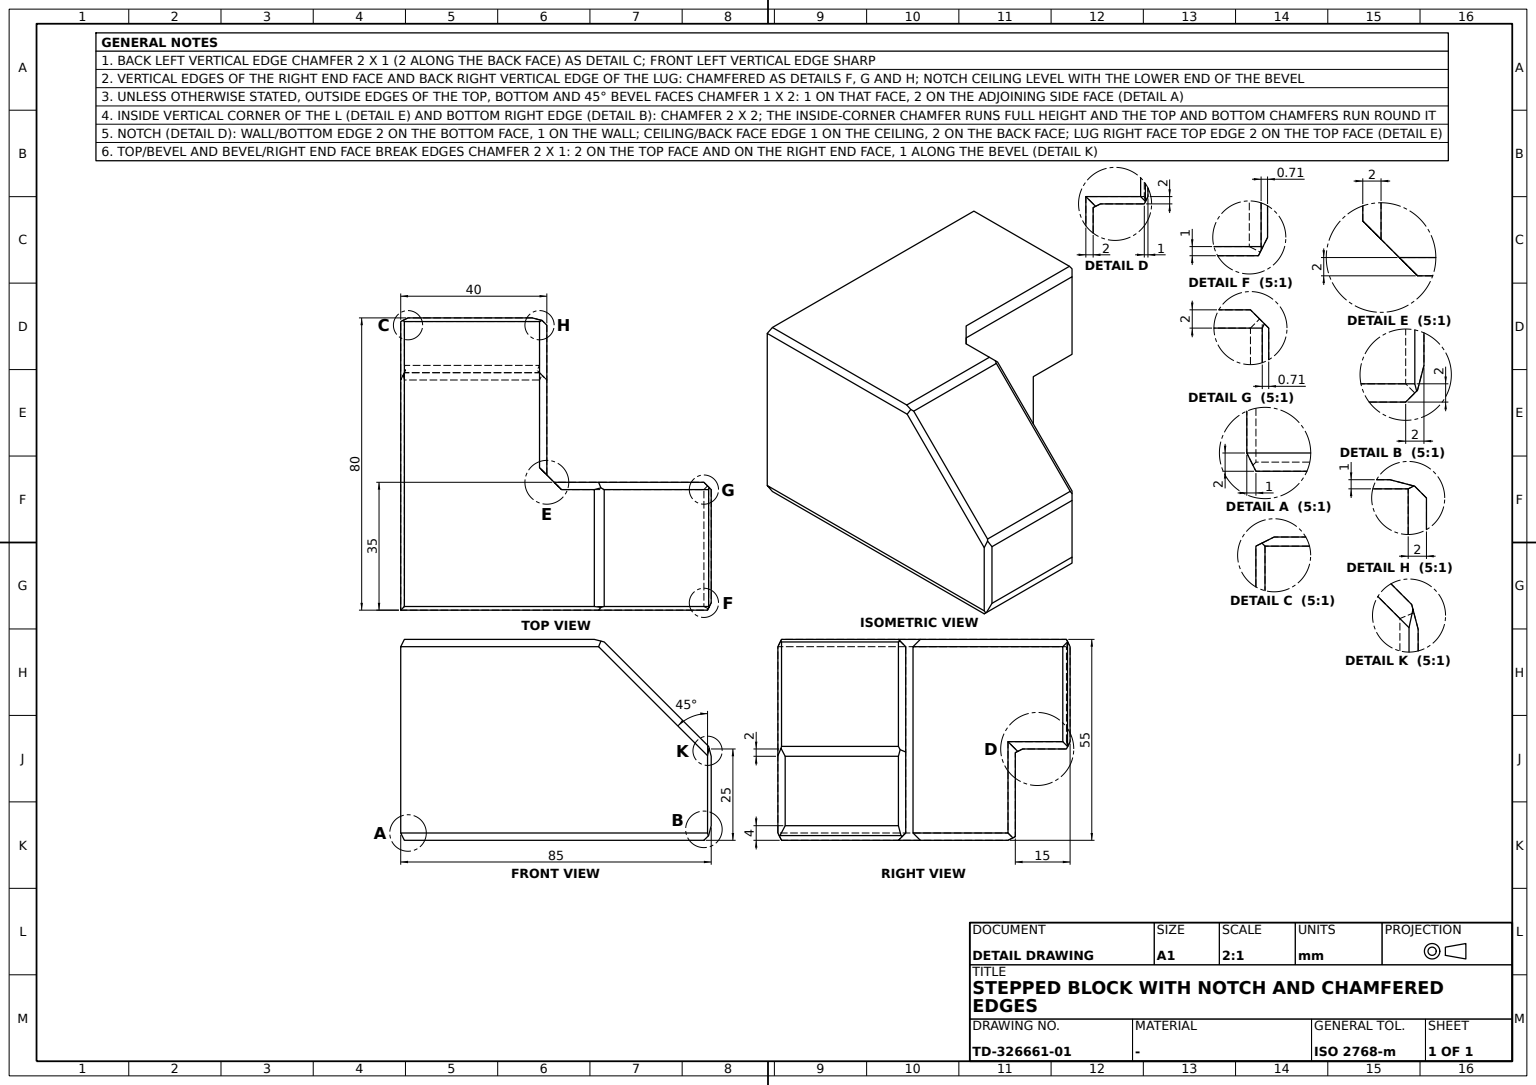
ISO-10303-21;
HEADER;
FILE_DESCRIPTION((''),'2;1');
FILE_NAME('','',(''),(''),'','','');
FILE_SCHEMA(('AUTOMOTIVE_DESIGN'));
ENDSEC;
DATA;
#1=APPLICATION_CONTEXT('');
#2=PRODUCT_CONTEXT('',#1,'mechanical');
#3=PRODUCT('','','',(#2));
#4=PRODUCT_DEFINITION_FORMATION('','',#3);
#5=PRODUCT_DEFINITION_CONTEXT('',#1,'design');
#6=PRODUCT_DEFINITION('','',#4,#5);
#7=PRODUCT_DEFINITION_SHAPE('','',#6);
#8=(LENGTH_UNIT()NAMED_UNIT(*)SI_UNIT(.MILLI.,.METRE.));
#9=(NAMED_UNIT(*)PLANE_ANGLE_UNIT()SI_UNIT($,.RADIAN.));
#10=(NAMED_UNIT(*)SI_UNIT($,.STERADIAN.)SOLID_ANGLE_UNIT());
#11=UNCERTAINTY_MEASURE_WITH_UNIT(LENGTH_MEASURE(0.005),#8,'distance_accuracy_value','');
#12=(GEOMETRIC_REPRESENTATION_CONTEXT(3)GLOBAL_UNCERTAINTY_ASSIGNED_CONTEXT((#11))GLOBAL_UNIT_ASSIGNED_CONTEXT((#8,#9,#10))REPRESENTATION_CONTEXT('',''));
#13=CARTESIAN_POINT('',(-42.5,-80.,53.));
#14=VERTEX_POINT('',#13);
#15=CARTESIAN_POINT('',(-41.5,-79.,55.));
#16=VERTEX_POINT('',#15);
#17=CARTESIAN_POINT('',(-45.166667,-82.666667,47.666667));
#18=DIRECTION('',(0.40824829,0.40824829,0.816496581));
#19=VECTOR('',#18,1000.);
#20=LINE('',#17,#19);
#21=EDGE_CURVE('',#14,#16,#20,.T.);
#22=ORIENTED_EDGE('',*,*,#21,.T.);
#23=CARTESIAN_POINT('',(-41.5,-1.,55.));
#24=VERTEX_POINT('',#23);
#25=CARTESIAN_POINT('',(-41.5,0.,55.));
#26=DIRECTION('',(0.,1.,0.));
#27=VECTOR('',#26,1000.);
#28=LINE('',#25,#27);
#29=EDGE_CURVE('',#16,#24,#28,.T.);
#30=ORIENTED_EDGE('',*,*,#29,.T.);
#31=CARTESIAN_POINT('',(-41.833333,-0.666667,54.333333));
#32=VERTEX_POINT('',#31);
#33=CARTESIAN_POINT('',(-44.066667,1.566667,49.866667));
#34=DIRECTION('',(0.40824829,-0.40824829,0.816496581));
#35=VECTOR('',#34,1000.);
#36=LINE('',#33,#35);
#37=EDGE_CURVE('',#32,#24,#36,.T.);
#38=ORIENTED_EDGE('',*,*,#37,.F.);
#39=CARTESIAN_POINT('',(-42.5,-1.,53.));
#40=VERTEX_POINT('',#39);
#41=CARTESIAN_POINT('',(-66.252381,-12.87619,5.495238));
#42=DIRECTION('',(0.43643578,0.21821789,0.872871561));
#43=VECTOR('',#42,1000.);
#44=LINE('',#41,#43);
#45=EDGE_CURVE('',#40,#32,#44,.T.);
#46=ORIENTED_EDGE('',*,*,#45,.F.);
#47=CARTESIAN_POINT('',(-42.5,-96.,53.));
#48=LINE('',#47,#27);
#49=EDGE_CURVE('',#14,#40,#48,.T.);
#50=ORIENTED_EDGE('',*,*,#49,.F.);
#51=EDGE_LOOP('',(#22,#30,#38,#46,#50));
#52=FACE_BOUND('',#51,.T.);
#53=DIRECTION('',(0.894427191,0.,-0.447213595));
#54=AXIS2_PLACEMENT_3D('',#47,#53,#26);
#55=PLANE('',#54);
#56=ADVANCED_FACE('',(#52),#55,.F.);
#57=CARTESIAN_POINT('',(13.207107,-47.,54.292893));
#58=VERTEX_POINT('',#57);
#59=CARTESIAN_POINT('',(13.207107,-79.,54.292893));
#60=VERTEX_POINT('',#59);
#61=CARTESIAN_POINT('',(13.207107,16.,54.292893));
#62=DIRECTION('',(0.,-1.,0.));
#63=VECTOR('',#62,1000.);
#64=LINE('',#61,#63);
#65=EDGE_CURVE('',#58,#60,#64,.T.);
#66=ORIENTED_EDGE('',*,*,#65,.F.);
#67=CARTESIAN_POINT('',(12.304738,-46.528595,54.528595));
#68=VERTEX_POINT('',#67);
#69=CARTESIAN_POINT('',(-13.48926,-33.053611,61.266088));
#70=DIRECTION('',(-0.863502056,0.451100166,0.225550083));
#71=VECTOR('',#70,1000.);
#72=LINE('',#69,#71);
#73=EDGE_CURVE('',#58,#68,#72,.T.);
#74=ORIENTED_EDGE('',*,*,#73,.T.);
#75=CARTESIAN_POINT('',(10.5,-47.,55.));
#76=VERTEX_POINT('',#75);
#77=CARTESIAN_POINT('',(24.97998,-43.217773,51.217773));
#78=DIRECTION('',(0.938045473,0.245021112,-0.245021112));
#79=VECTOR('',#78,1000.);
#80=LINE('',#77,#79);
#81=EDGE_CURVE('',#76,#68,#80,.T.);
#82=ORIENTED_EDGE('',*,*,#81,.F.);
#83=CARTESIAN_POINT('',(10.5,-79.,55.));
#84=VERTEX_POINT('',#83);
#85=CARTESIAN_POINT('',(10.5,16.,55.));
#86=LINE('',#85,#63);
#87=EDGE_CURVE('',#76,#84,#86,.T.);
#88=ORIENTED_EDGE('',*,*,#87,.T.);
#89=CARTESIAN_POINT('',(12.304738,-79.235702,54.528595));
#90=VERTEX_POINT('',#89);
#91=CARTESIAN_POINT('',(55.145452,-84.830783,43.338435));
#92=DIRECTION('',(0.959904955,-0.125365447,-0.250730894));
#93=VECTOR('',#92,1000.);
#94=LINE('',#91,#93);
#95=EDGE_CURVE('',#84,#90,#94,.T.);
#96=ORIENTED_EDGE('',*,*,#95,.T.);
#97=CARTESIAN_POINT('',(-2.503749,-83.103736,58.39663));
#98=DIRECTION('',(-0.938045473,-0.245021112,0.245021112));
#99=VECTOR('',#98,1000.);
#100=LINE('',#97,#99);
#101=EDGE_CURVE('',#60,#90,#100,.T.);
#102=ORIENTED_EDGE('',*,*,#101,.F.);
#103=EDGE_LOOP('',(#66,#74,#82,#88,#96,#102));
#104=FACE_BOUND('',#103,.T.);
#105=DIRECTION('',(0.252724733,0.,0.967538221));
#106=AXIS2_PLACEMENT_3D('',#85,#105,#62);
#107=PLANE('',#106);
#108=ADVANCED_FACE('',(#104),#107,.T.);
#109=CARTESIAN_POINT('',(-41.5,-17.,0.));
#110=VERTEX_POINT('',#109);
#111=CARTESIAN_POINT('',(-41.833333,-15.666667,0.666667));
#112=VERTEX_POINT('',#111);
#113=CARTESIAN_POINT('',(-36.804762,-35.780952,-9.390476));
#114=DIRECTION('',(-0.21821789,0.872871561,0.43643578));
#115=VECTOR('',#114,1000.);
#116=LINE('',#113,#115);
#117=EDGE_CURVE('',#110,#112,#116,.T.);
#118=ORIENTED_EDGE('',*,*,#117,.F.);
#119=CARTESIAN_POINT('',(-41.5,-79.,0.));
#120=VERTEX_POINT('',#119);
#121=CARTESIAN_POINT('',(-41.5,-95.8,0.));
#122=LINE('',#121,#27);
#123=EDGE_CURVE('',#120,#110,#122,.T.);
#124=ORIENTED_EDGE('',*,*,#123,.F.);
#125=CARTESIAN_POINT('',(-42.5,-80.,2.));
#126=VERTEX_POINT('',#125);
#127=CARTESIAN_POINT('',(-45.133333,-82.633333,7.266667));
#128=DIRECTION('',(-0.40824829,-0.40824829,0.816496581));
#129=VECTOR('',#128,1000.);
#130=LINE('',#127,#129);
#131=EDGE_CURVE('',#120,#126,#130,.T.);
#132=ORIENTED_EDGE('',*,*,#131,.T.);
#133=CARTESIAN_POINT('',(-42.5,-17.,2.));
#134=VERTEX_POINT('',#133);
#135=CARTESIAN_POINT('',(-42.5,-95.8,2.));
#136=LINE('',#135,#27);
#137=EDGE_CURVE('',#126,#134,#136,.T.);
#138=ORIENTED_EDGE('',*,*,#137,.T.);
#139=CARTESIAN_POINT('',(-60.011111,-52.022222,37.022222));
#140=DIRECTION('',(-0.333333333,-0.666666667,0.666666667));
#141=VECTOR('',#140,1000.);
#142=LINE('',#139,#141);
#143=EDGE_CURVE('',#112,#134,#142,.T.);
#144=ORIENTED_EDGE('',*,*,#143,.F.);
#145=EDGE_LOOP('',(#118,#124,#132,#138,#144));
#146=FACE_BOUND('',#145,.T.);
#147=DIRECTION('',(-0.894427191,0.,-0.447213595));
#148=AXIS2_PLACEMENT_3D('',#135,#147,#26);
#149=PLANE('',#148);
#150=ADVANCED_FACE('',(#146),#149,.T.);
#151=CARTESIAN_POINT('',(-41.833333,-0.666667,25.666667));
#152=VERTEX_POINT('',#151);
#153=CARTESIAN_POINT('',(-41.5,-1.,25.));
#154=VERTEX_POINT('',#153);
#155=CARTESIAN_POINT('',(-26.533333,-15.966667,-4.933333));
#156=DIRECTION('',(0.40824829,-0.40824829,-0.816496581));
#157=VECTOR('',#156,1000.);
#158=LINE('',#155,#157);
#159=EDGE_CURVE('',#152,#154,#158,.T.);
#160=ORIENTED_EDGE('',*,*,#159,.T.);
#161=CARTESIAN_POINT('',(-41.5,-13.,25.));
#162=VERTEX_POINT('',#161);
#163=CARTESIAN_POINT('',(-41.5,-95.8,25.));
#164=LINE('',#163,#27);
#165=EDGE_CURVE('',#162,#154,#164,.T.);
#166=ORIENTED_EDGE('',*,*,#165,.F.);
#167=CARTESIAN_POINT('',(-41.166667,-14.333333,24.333333));
#168=VERTEX_POINT('',#167);
#169=CARTESIAN_POINT('',(-25.966667,-75.133333,-6.066667));
#170=LINE('',#169,#115);
#171=EDGE_CURVE('',#168,#162,#170,.T.);
#172=ORIENTED_EDGE('',*,*,#171,.F.);
#173=CARTESIAN_POINT('',(-42.5,-17.,27.));
#174=VERTEX_POINT('',#173);
#175=CARTESIAN_POINT('',(-60.011111,-52.022222,62.022222));
#176=LINE('',#175,#141);
#177=EDGE_CURVE('',#168,#174,#176,.T.);
#178=ORIENTED_EDGE('',*,*,#177,.T.);
#179=CARTESIAN_POINT('',(-42.5,-1.,27.));
#180=VERTEX_POINT('',#179);
#181=CARTESIAN_POINT('',(-42.5,-95.8,27.));
#182=LINE('',#181,#27);
#183=EDGE_CURVE('',#174,#180,#182,.T.);
#184=ORIENTED_EDGE('',*,*,#183,.T.);
#185=CARTESIAN_POINT('',(-51.528571,-5.514286,45.057143));
#186=DIRECTION('',(-0.43643578,-0.21821789,0.872871561));
#187=VECTOR('',#186,1000.);
#188=LINE('',#185,#187);
#189=EDGE_CURVE('',#152,#180,#188,.T.);
#190=ORIENTED_EDGE('',*,*,#189,.F.);
#191=EDGE_LOOP('',(#160,#166,#172,#178,#184,#190));
#192=FACE_BOUND('',#191,.T.);
#193=AXIS2_PLACEMENT_3D('',#181,#147,#26);
#194=PLANE('',#193);
#195=ADVANCED_FACE('',(#192),#194,.T.);
#196=CARTESIAN_POINT('',(-40.5,0.,53.));
#197=VERTEX_POINT('',#196);
#198=CARTESIAN_POINT('',(-6.5,0.,53.));
#199=VERTEX_POINT('',#198);
#200=CARTESIAN_POINT('',(-51.9,0.,53.));
#201=DIRECTION('',(1.,0.,0.));
#202=VECTOR('',#201,1000.);
#203=LINE('',#200,#202);
#204=EDGE_CURVE('',#197,#199,#203,.T.);
#205=ORIENTED_EDGE('',*,*,#204,.T.);
#206=CARTESIAN_POINT('',(-6.5,0.,27.));
#207=VERTEX_POINT('',#206);
#208=CARTESIAN_POINT('',(-6.5,0.,19.933333));
#209=DIRECTION('',(0.,0.,1.));
#210=VECTOR('',#209,1000.);
#211=LINE('',#208,#210);
#212=EDGE_CURVE('',#207,#199,#211,.T.);
#213=ORIENTED_EDGE('',*,*,#212,.F.);
#214=CARTESIAN_POINT('',(-40.5,0.,27.));
#215=VERTEX_POINT('',#214);
#216=CARTESIAN_POINT('',(-50.1,0.,27.));
#217=LINE('',#216,#202);
#218=EDGE_CURVE('',#215,#207,#217,.T.);
#219=ORIENTED_EDGE('',*,*,#218,.F.);
#220=CARTESIAN_POINT('',(-40.5,0.,-10.6));
#221=LINE('',#220,#210);
#222=EDGE_CURVE('',#215,#197,#221,.T.);
#223=ORIENTED_EDGE('',*,*,#222,.T.);
#224=EDGE_LOOP('',(#205,#213,#219,#223));
#225=FACE_BOUND('',#224,.T.);
#226=CARTESIAN_POINT('',(-2.5,0.,0.));
#227=DIRECTION('',(-1.,0.,0.));
#228=AXIS2_PLACEMENT_3D('',#226,#26,#227);
#229=PLANE('',#228);
#230=ADVANCED_FACE('',(#225),#229,.T.);
#231=CARTESIAN_POINT('',(-41.5,-15.,24.));
#232=VERTEX_POINT('',#231);
#233=CARTESIAN_POINT('',(-33.266667,1.466667,32.233333));
#234=DIRECTION('',(0.40824829,0.816496581,0.40824829));
#235=VECTOR('',#234,1000.);
#236=LINE('',#233,#235);
#237=EDGE_CURVE('',#232,#168,#236,.T.);
#238=ORIENTED_EDGE('',*,*,#237,.T.);
#239=ORIENTED_EDGE('',*,*,#171,.T.);
#240=CARTESIAN_POINT('',(-4.5,-13.,25.));
#241=VERTEX_POINT('',#240);
#242=CARTESIAN_POINT('',(2.9,-13.,25.));
#243=VECTOR('',#227,1000.);
#244=LINE('',#242,#243);
#245=EDGE_CURVE('',#241,#162,#244,.T.);
#246=ORIENTED_EDGE('',*,*,#245,.F.);
#247=CARTESIAN_POINT('',(-5.166667,-14.333333,24.333333));
#248=VERTEX_POINT('',#247);
#249=CARTESIAN_POINT('',(-3.266667,-10.533333,26.233333));
#250=LINE('',#249,#235);
#251=EDGE_CURVE('',#248,#241,#250,.T.);
#252=ORIENTED_EDGE('',*,*,#251,.F.);
#253=CARTESIAN_POINT('',(-4.5,-15.,24.));
#254=VERTEX_POINT('',#253);
#255=CARTESIAN_POINT('',(-13.3,-6.2,28.4));
#256=DIRECTION('',(-0.666666667,0.666666667,0.333333333));
#257=VECTOR('',#256,1000.);
#258=LINE('',#255,#257);
#259=EDGE_CURVE('',#254,#248,#258,.T.);
#260=ORIENTED_EDGE('',*,*,#259,.F.);
#261=CARTESIAN_POINT('',(2.9,-15.,24.));
#262=LINE('',#261,#243);
#263=EDGE_CURVE('',#254,#232,#262,.T.);
#264=ORIENTED_EDGE('',*,*,#263,.T.);
#265=EDGE_LOOP('',(#238,#239,#246,#252,#260,#264));
#266=FACE_BOUND('',#265,.T.);
#267=DIRECTION('',(0.,-0.447213595,0.894427191));
#268=AXIS2_PLACEMENT_3D('',#242,#267,#227);
#269=PLANE('',#268);
#270=ADVANCED_FACE('',(#266),#269,.F.);
#271=CARTESIAN_POINT('',(-2.5,-2.,53.));
#272=VERTEX_POINT('',#271);
#273=CARTESIAN_POINT('',(-2.5,-43.,53.));
#274=VERTEX_POINT('',#273);
#275=CARTESIAN_POINT('',(-2.5,16.,53.));
#276=LINE('',#275,#63);
#277=EDGE_CURVE('',#272,#274,#276,.T.);
#278=ORIENTED_EDGE('',*,*,#277,.T.);
#279=CARTESIAN_POINT('',(-2.5,-43.,2.));
#280=VERTEX_POINT('',#279);
#281=CARTESIAN_POINT('',(-2.5,-43.,0.));
#282=LINE('',#281,#210);
#283=EDGE_CURVE('',#280,#274,#282,.T.);
#284=ORIENTED_EDGE('',*,*,#283,.F.);
#285=CARTESIAN_POINT('',(-2.5,-17.,2.));
#286=VERTEX_POINT('',#285);
#287=CARTESIAN_POINT('',(-2.5,-45.,2.));
#288=LINE('',#287,#27);
#289=EDGE_CURVE('',#280,#286,#288,.T.);
#290=ORIENTED_EDGE('',*,*,#289,.T.);
#291=CARTESIAN_POINT('',(-2.5,-17.,27.));
#292=VERTEX_POINT('',#291);
#293=CARTESIAN_POINT('',(-2.5,-17.,0.));
#294=DIRECTION('',(0.,0.,-1.));
#295=VECTOR('',#294,1000.);
#296=LINE('',#293,#295);
#297=EDGE_CURVE('',#292,#286,#296,.T.);
#298=ORIENTED_EDGE('',*,*,#297,.F.);
#299=CARTESIAN_POINT('',(-2.5,-2.,27.));
#300=VERTEX_POINT('',#299);
#301=CARTESIAN_POINT('',(-2.5,-45.,27.));
#302=LINE('',#301,#27);
#303=EDGE_CURVE('',#292,#300,#302,.T.);
#304=ORIENTED_EDGE('',*,*,#303,.T.);
#305=CARTESIAN_POINT('',(-2.5,-2.,0.));
#306=LINE('',#305,#295);
#307=EDGE_CURVE('',#272,#300,#306,.T.);
#308=ORIENTED_EDGE('',*,*,#307,.F.);
#309=EDGE_LOOP('',(#278,#284,#290,#298,#304,#308));
#310=FACE_BOUND('',#309,.T.);
#311=CARTESIAN_POINT('',(-2.5,-45.,0.));
#312=AXIS2_PLACEMENT_3D('',#311,#201,#26);
#313=PLANE('',#312);
#314=ADVANCED_FACE('',(#310),#313,.T.);
#315=CARTESIAN_POINT('',(-4.5,-41.,55.));
#316=VERTEX_POINT('',#315);
#317=CARTESIAN_POINT('',(1.5,-47.,55.));
#318=VERTEX_POINT('',#317);
#319=CARTESIAN_POINT('',(-2.5,-43.,55.));
#320=DIRECTION('',(0.707106781,-0.707106781,0.));
#321=VECTOR('',#320,1000.);
#322=LINE('',#319,#321);
#323=EDGE_CURVE('',#316,#318,#322,.T.);
#324=ORIENTED_EDGE('',*,*,#323,.F.);
#325=CARTESIAN_POINT('',(-4.5,-1.,55.));
#326=VERTEX_POINT('',#325);
#327=CARTESIAN_POINT('',(-4.5,0.,55.));
#328=LINE('',#327,#63);
#329=EDGE_CURVE('',#326,#316,#328,.T.);
#330=ORIENTED_EDGE('',*,*,#329,.F.);
#331=CARTESIAN_POINT('',(0.,-1.,55.));
#332=LINE('',#331,#202);
#333=EDGE_CURVE('',#24,#326,#332,.T.);
#334=ORIENTED_EDGE('',*,*,#333,.F.);
#335=ORIENTED_EDGE('',*,*,#29,.F.);
#336=CARTESIAN_POINT('',(0.,-79.,55.));
#337=LINE('',#336,#243);
#338=EDGE_CURVE('',#84,#16,#337,.T.);
#339=ORIENTED_EDGE('',*,*,#338,.F.);
#340=ORIENTED_EDGE('',*,*,#87,.F.);
#341=CARTESIAN_POINT('',(0.,-47.,55.));
#342=LINE('',#341,#202);
#343=EDGE_CURVE('',#318,#76,#342,.T.);
#344=ORIENTED_EDGE('',*,*,#343,.F.);
#345=EDGE_LOOP('',(#324,#330,#334,#335,#339,#340,#344));
#346=FACE_BOUND('',#345,.T.);
#347=CARTESIAN_POINT('',(0.,0.,55.));
#348=AXIS2_PLACEMENT_3D('',#347,#209,#201);
#349=PLANE('',#348);
#350=ADVANCED_FACE('',(#346),#349,.T.);
#351=CARTESIAN_POINT('',(40.5,-79.,0.));
#352=VERTEX_POINT('',#351);
#353=CARTESIAN_POINT('',(40.5,-47.,0.));
#354=VERTEX_POINT('',#353);
#355=CARTESIAN_POINT('',(40.5,0.,0.));
#356=LINE('',#355,#27);
#357=EDGE_CURVE('',#352,#354,#356,.T.);
#358=ORIENTED_EDGE('',*,*,#357,.T.);
#359=CARTESIAN_POINT('',(41.5,-46.,1.));
#360=VERTEX_POINT('',#359);
#361=CARTESIAN_POINT('',(46.833333,-40.666667,6.333333));
#362=DIRECTION('',(-0.577350269,-0.577350269,-0.577350269));
#363=VECTOR('',#362,1000.);
#364=LINE('',#361,#363);
#365=EDGE_CURVE('',#360,#354,#364,.T.);
#366=ORIENTED_EDGE('',*,*,#365,.F.);
#367=CARTESIAN_POINT('',(41.792893,-46.292893,1.292893));
#368=VERTEX_POINT('',#367);
#369=CARTESIAN_POINT('',(62.366667,-66.866667,21.866667));
#370=DIRECTION('',(0.577350269,-0.577350269,0.577350269));
#371=VECTOR('',#370,1000.);
#372=LINE('',#369,#371);
#373=EDGE_CURVE('',#360,#368,#372,.T.);
#374=ORIENTED_EDGE('',*,*,#373,.T.);
#375=CARTESIAN_POINT('',(41.792893,-79.414214,1.292893));
#376=VERTEX_POINT('',#375);
#377=CARTESIAN_POINT('',(41.792893,-93.,1.292893));
#378=LINE('',#377,#27);
#379=EDGE_CURVE('',#376,#368,#378,.T.);
#380=ORIENTED_EDGE('',*,*,#379,.F.);
#381=CARTESIAN_POINT('',(41.7,-79.6,1.2));
#382=VERTEX_POINT('',#381);
#383=CARTESIAN_POINT('',(36.833333,-89.333333,-3.666667));
#384=LINE('',#383,#235);
#385=EDGE_CURVE('',#382,#376,#384,.T.);
#386=ORIENTED_EDGE('',*,*,#385,.F.);
#387=CARTESIAN_POINT('',(49.522222,-83.511111,9.022222));
#388=DIRECTION('',(0.666666667,-0.333333333,0.666666667));
#389=VECTOR('',#388,1000.);
#390=LINE('',#387,#389);
#391=EDGE_CURVE('',#352,#382,#390,.T.);
#392=ORIENTED_EDGE('',*,*,#391,.F.);
#393=EDGE_LOOP('',(#358,#366,#374,#380,#386,#392));
#394=FACE_BOUND('',#393,.T.);
#395=CARTESIAN_POINT('',(40.5,-93.,0.));
#396=DIRECTION('',(0.707106781,0.,-0.707106781));
#397=AXIS2_PLACEMENT_3D('',#395,#396,#26);
#398=PLANE('',#397);
#399=ADVANCED_FACE('',(#394),#398,.T.);
#400=CARTESIAN_POINT('',(1.5,-47.,0.));
#401=VERTEX_POINT('',#400);
#402=CARTESIAN_POINT('',(0.,-47.,0.));
#403=LINE('',#402,#243);
#404=EDGE_CURVE('',#354,#401,#403,.T.);
#405=ORIENTED_EDGE('',*,*,#404,.F.);
#406=ORIENTED_EDGE('',*,*,#357,.F.);
#407=CARTESIAN_POINT('',(58.3,-79.,0.));
#408=LINE('',#407,#243);
#409=EDGE_CURVE('',#352,#120,#408,.T.);
#410=ORIENTED_EDGE('',*,*,#409,.T.);
#411=ORIENTED_EDGE('',*,*,#123,.T.);
#412=CARTESIAN_POINT('',(-4.5,-17.,0.));
#413=VERTEX_POINT('',#412);
#414=CARTESIAN_POINT('',(0.,-17.,0.));
#415=LINE('',#414,#243);
#416=EDGE_CURVE('',#413,#110,#415,.T.);
#417=ORIENTED_EDGE('',*,*,#416,.F.);
#418=CARTESIAN_POINT('',(-4.5,-41.,0.));
#419=VERTEX_POINT('',#418);
#420=CARTESIAN_POINT('',(-4.5,0.,0.));
#421=LINE('',#420,#27);
#422=EDGE_CURVE('',#419,#413,#421,.T.);
#423=ORIENTED_EDGE('',*,*,#422,.F.);
#424=LINE('',#281,#321);
#425=EDGE_CURVE('',#419,#401,#424,.T.);
#426=ORIENTED_EDGE('',*,*,#425,.T.);
#427=EDGE_LOOP('',(#405,#406,#410,#411,#417,#423,#426));
#428=FACE_BOUND('',#427,.T.);
#429=CARTESIAN_POINT('',(0.,0.,0.));
#430=AXIS2_PLACEMENT_3D('',#429,#209,#201);
#431=PLANE('',#430);
#432=ADVANCED_FACE('',(#428),#431,.F.);
#433=CARTESIAN_POINT('',(42.5,-78.,23.));
#434=VERTEX_POINT('',#433);
#435=CARTESIAN_POINT('',(42.5,-78.,4.));
#436=VERTEX_POINT('',#435);
#437=CARTESIAN_POINT('',(42.5,-78.,66.));
#438=LINE('',#437,#295);
#439=EDGE_CURVE('',#434,#436,#438,.T.);
#440=ORIENTED_EDGE('',*,*,#439,.F.);
#441=CARTESIAN_POINT('',(41.930964,-79.138071,25.178511));
#442=VERTEX_POINT('',#441);
#443=CARTESIAN_POINT('',(41.624987,-79.750026,26.349923));
#444=DIRECTION('',(-0.225550083,-0.451100166,0.863502056));
#445=VECTOR('',#444,1000.);
#446=LINE('',#443,#445);
#447=EDGE_CURVE('',#434,#442,#446,.T.);
#448=ORIENTED_EDGE('',*,*,#447,.T.);
#449=CARTESIAN_POINT('',(41.5,-80.,23.171573));
#450=VERTEX_POINT('',#449);
#451=CARTESIAN_POINT('',(49.161077,-64.677845,58.848093));
#452=DIRECTION('',(0.19357795,0.387155901,0.901464301));
#453=VECTOR('',#452,1000.);
#454=LINE('',#451,#453);
#455=EDGE_CURVE('',#450,#442,#454,.T.);
#456=ORIENTED_EDGE('',*,*,#455,.F.);
#457=CARTESIAN_POINT('',(41.5,-80.,2.));
#458=VERTEX_POINT('',#457);
#459=CARTESIAN_POINT('',(41.5,-80.,0.));
#460=LINE('',#459,#295);
#461=EDGE_CURVE('',#450,#458,#460,.T.);
#462=ORIENTED_EDGE('',*,*,#461,.T.);
#463=CARTESIAN_POINT('',(42.3,-78.4,-1.2));
#464=DIRECTION('',(0.21821789,0.43643578,-0.872871561));
#465=VECTOR('',#464,1000.);
#466=LINE('',#463,#465);
#467=EDGE_CURVE('',#458,#382,#466,.T.);
#468=ORIENTED_EDGE('',*,*,#467,.T.);
#469=ORIENTED_EDGE('',*,*,#385,.T.);
#470=CARTESIAN_POINT('',(41.604638,-79.790724,0.572172));
#471=DIRECTION('',(-0.225550083,-0.451100166,-0.863502056));
#472=VECTOR('',#471,1000.);
#473=LINE('',#470,#472);
#474=EDGE_CURVE('',#436,#376,#473,.T.);
#475=ORIENTED_EDGE('',*,*,#474,.F.);
#476=EDGE_LOOP('',(#440,#448,#456,#462,#468,#469,#475));
#477=FACE_BOUND('',#476,.T.);
#478=DIRECTION('',(-0.894427191,0.447213595,0.));
#479=AXIS2_PLACEMENT_3D('',#437,#478,#294);
#480=PLANE('',#479);
#481=ADVANCED_FACE('',(#477),#480,.F.);
#482=CARTESIAN_POINT('',(41.792893,-79.,25.707107));
#483=VERTEX_POINT('',#482);
#484=CARTESIAN_POINT('',(42.913817,-80.120924,21.415731));
#485=DIRECTION('',(0.245021112,-0.245021112,-0.938045473));
#486=VECTOR('',#485,1000.);
#487=LINE('',#484,#486);
#488=EDGE_CURVE('',#483,#442,#487,.T.);
#489=ORIENTED_EDGE('',*,*,#488,.F.);
#490=CARTESIAN_POINT('',(0.085786,-79.,67.414214));
#491=VECTOR('',#396,1000.);
#492=LINE('',#490,#491);
#493=EDGE_CURVE('',#60,#483,#492,.T.);
#494=ORIENTED_EDGE('',*,*,#493,.F.);
#495=ORIENTED_EDGE('',*,*,#101,.T.);
#496=CARTESIAN_POINT('',(11.671573,-80.,53.));
#497=VERTEX_POINT('',#496);
#498=CARTESIAN_POINT('',(17.299264,-73.206776,66.586449));
#499=DIRECTION('',(-0.347407948,-0.41935849,-0.838716981));
#500=VECTOR('',#499,1000.);
#501=LINE('',#498,#500);
#502=EDGE_CURVE('',#90,#497,#501,.T.);
#503=ORIENTED_EDGE('',*,*,#502,.T.);
#504=CARTESIAN_POINT('',(-1.328427,-80.,66.));
#505=LINE('',#504,#491);
#506=EDGE_CURVE('',#497,#450,#505,.T.);
#507=ORIENTED_EDGE('',*,*,#506,.T.);
#508=ORIENTED_EDGE('',*,*,#455,.T.);
#509=EDGE_LOOP('',(#489,#494,#495,#503,#507,#508));
#510=FACE_BOUND('',#509,.T.);
#511=DIRECTION('',(0.316227766,-0.894427191,0.316227766));
#512=AXIS2_PLACEMENT_3D('',#504,#511,#396);
#513=PLANE('',#512);
#514=ADVANCED_FACE('',(#510),#513,.T.);
#515=CARTESIAN_POINT('',(41.792893,-47.,25.707107));
#516=VERTEX_POINT('',#515);
#517=CARTESIAN_POINT('',(50.114214,-47.,17.385786));
#518=DIRECTION('',(-0.707106781,0.,0.707106781));
#519=VECTOR('',#518,1000.);
#520=LINE('',#517,#519);
#521=EDGE_CURVE('',#516,#58,#520,.T.);
#522=ORIENTED_EDGE('',*,*,#521,.T.);
#523=ORIENTED_EDGE('',*,*,#65,.T.);
#524=ORIENTED_EDGE('',*,*,#493,.T.);
#525=CARTESIAN_POINT('',(41.792893,-86.6,25.707107));
#526=LINE('',#525,#27);
#527=EDGE_CURVE('',#483,#516,#526,.T.);
#528=ORIENTED_EDGE('',*,*,#527,.T.);
#529=EDGE_LOOP('',(#522,#523,#524,#528));
#530=FACE_BOUND('',#529,.T.);
#531=CARTESIAN_POINT('',(42.5,16.,25.));
#532=DIRECTION('',(-0.707106781,0.,-0.707106781));
#533=AXIS2_PLACEMENT_3D('',#531,#532,#62);
#534=PLANE('',#533);
#535=ADVANCED_FACE('',(#530),#534,.F.);
#536=ORIENTED_EDGE('',*,*,#289,.F.);
#537=CARTESIAN_POINT('',(-6.833333,-38.666667,-2.333333));
#538=DIRECTION('',(-0.577350269,0.577350269,-0.577350269));
#539=VECTOR('',#538,1000.);
#540=LINE('',#537,#539);
#541=EDGE_CURVE('',#280,#419,#540,.T.);
#542=ORIENTED_EDGE('',*,*,#541,.T.);
#543=ORIENTED_EDGE('',*,*,#422,.T.);
#544=CARTESIAN_POINT('',(-3.833333,-15.666667,0.666667));
#545=VERTEX_POINT('',#544);
#546=CARTESIAN_POINT('',(5.766667,3.533333,10.266667));
#547=DIRECTION('',(-0.40824829,-0.816496581,-0.40824829));
#548=VECTOR('',#547,1000.);
#549=LINE('',#546,#548);
#550=EDGE_CURVE('',#545,#413,#549,.T.);
#551=ORIENTED_EDGE('',*,*,#550,.F.);
#552=CARTESIAN_POINT('',(16.7,-36.2,21.2));
#553=LINE('',#552,#371);
#554=EDGE_CURVE('',#545,#286,#553,.T.);
#555=ORIENTED_EDGE('',*,*,#554,.T.);
#556=EDGE_LOOP('',(#536,#542,#543,#551,#555));
#557=FACE_BOUND('',#556,.T.);
#558=CARTESIAN_POINT('',(-4.5,-93.,0.));
#559=AXIS2_PLACEMENT_3D('',#558,#396,#26);
#560=PLANE('',#559);
#561=ADVANCED_FACE('',(#557),#560,.T.);
#562=ORIENTED_EDGE('',*,*,#165,.T.);
#563=CARTESIAN_POINT('',(-4.5,-1.,25.));
#564=VERTEX_POINT('',#563);
#565=CARTESIAN_POINT('',(-50.1,-1.,25.));
#566=LINE('',#565,#202);
#567=EDGE_CURVE('',#154,#564,#566,.T.);
#568=ORIENTED_EDGE('',*,*,#567,.T.);
#569=CARTESIAN_POINT('',(-4.5,-15.,25.));
#570=LINE('',#569,#27);
#571=EDGE_CURVE('',#241,#564,#570,.T.);
#572=ORIENTED_EDGE('',*,*,#571,.F.);
#573=ORIENTED_EDGE('',*,*,#245,.T.);
#574=EDGE_LOOP('',(#562,#568,#572,#573));
#575=FACE_BOUND('',#574,.T.);
#576=CARTESIAN_POINT('',(-2.5,-15.,25.));
#577=AXIS2_PLACEMENT_3D('',#576,#209,#26);
#578=PLANE('',#577);
#579=ADVANCED_FACE('',(#575),#578,.F.);
#580=CARTESIAN_POINT('',(40.5,-45.,2.));
#581=VERTEX_POINT('',#580);
#582=CARTESIAN_POINT('',(48.166667,-52.666667,-5.666667));
#583=DIRECTION('',(-0.577350269,0.577350269,0.577350269));
#584=VECTOR('',#583,1000.);
#585=LINE('',#582,#584);
#586=EDGE_CURVE('',#360,#581,#585,.T.);
#587=ORIENTED_EDGE('',*,*,#586,.F.);
#588=ORIENTED_EDGE('',*,*,#365,.T.);
#589=ORIENTED_EDGE('',*,*,#404,.T.);
#590=CARTESIAN_POINT('',(-0.5,-45.,2.));
#591=VERTEX_POINT('',#590);
#592=CARTESIAN_POINT('',(20.833333,-66.333333,-19.333333));
#593=DIRECTION('',(0.577350269,-0.577350269,-0.577350269));
#594=VECTOR('',#593,1000.);
#595=LINE('',#592,#594);
#596=EDGE_CURVE('',#591,#401,#595,.T.);
#597=ORIENTED_EDGE('',*,*,#596,.F.);
#598=CARTESIAN_POINT('',(42.5,-45.,2.));
#599=LINE('',#598,#243);
#600=EDGE_CURVE('',#581,#591,#599,.T.);
#601=ORIENTED_EDGE('',*,*,#600,.F.);
#602=EDGE_LOOP('',(#587,#588,#589,#597,#601));
#603=FACE_BOUND('',#602,.T.);
#604=CARTESIAN_POINT('',(59.5,-47.,0.));
#605=DIRECTION('',(0.,0.707106781,-0.707106781));
#606=AXIS2_PLACEMENT_3D('',#604,#605,#227);
#607=PLANE('',#606);
#608=ADVANCED_FACE('',(#603),#607,.T.);
#609=ORIENTED_EDGE('',*,*,#461,.F.);
#610=ORIENTED_EDGE('',*,*,#506,.F.);
#611=CARTESIAN_POINT('',(58.3,-80.,53.));
#612=LINE('',#611,#243);
#613=EDGE_CURVE('',#497,#14,#612,.T.);
#614=ORIENTED_EDGE('',*,*,#613,.T.);
#615=CARTESIAN_POINT('',(-42.5,-80.,0.));
#616=LINE('',#615,#210);
#617=EDGE_CURVE('',#126,#14,#616,.T.);
#618=ORIENTED_EDGE('',*,*,#617,.F.);
#619=CARTESIAN_POINT('',(58.3,-80.,2.));
#620=LINE('',#619,#243);
#621=EDGE_CURVE('',#458,#126,#620,.T.);
#622=ORIENTED_EDGE('',*,*,#621,.F.);
#623=EDGE_LOOP('',(#609,#610,#614,#618,#622));
#624=FACE_BOUND('',#623,.T.);
#625=AXIS2_PLACEMENT_3D('',#615,#62,#201);
#626=PLANE('',#625);
#627=ADVANCED_FACE('',(#624),#626,.T.);
#628=ORIENTED_EDGE('',*,*,#259,.T.);
#629=CARTESIAN_POINT('',(7.7,-27.2,37.2));
#630=LINE('',#629,#539);
#631=EDGE_CURVE('',#292,#248,#630,.T.);
#632=ORIENTED_EDGE('',*,*,#631,.F.);
#633=ORIENTED_EDGE('',*,*,#297,.T.);
#634=ORIENTED_EDGE('',*,*,#554,.F.);
#635=CARTESIAN_POINT('',(-4.5,-15.,1.));
#636=VERTEX_POINT('',#635);
#637=CARTESIAN_POINT('',(23.988889,-43.488889,-13.244444));
#638=LINE('',#637,#257);
#639=EDGE_CURVE('',#545,#636,#638,.T.);
#640=ORIENTED_EDGE('',*,*,#639,.T.);
#641=CARTESIAN_POINT('',(-4.5,-15.,63.6));
#642=LINE('',#641,#295);
#643=EDGE_CURVE('',#254,#636,#642,.T.);
#644=ORIENTED_EDGE('',*,*,#643,.F.);
#645=EDGE_LOOP('',(#628,#632,#633,#634,#640,#644));
#646=FACE_BOUND('',#645,.T.);
#647=DIRECTION('',(-0.707106781,-0.707106781,0.));
#648=AXIS2_PLACEMENT_3D('',#641,#647,#294);
#649=PLANE('',#648);
#650=ADVANCED_FACE('',(#646),#649,.F.);
#651=ORIENTED_EDGE('',*,*,#333,.T.);
#652=CARTESIAN_POINT('',(-3.872583,-0.686292,54.372583));
#653=VERTEX_POINT('',#652);
#654=CARTESIAN_POINT('',(1.055556,1.777778,49.444444));
#655=DIRECTION('',(-0.666666667,-0.333333333,0.666666667));
#656=VECTOR('',#655,1000.);
#657=LINE('',#654,#656);
#658=EDGE_CURVE('',#653,#326,#657,.T.);
#659=ORIENTED_EDGE('',*,*,#658,.F.);
#660=CARTESIAN_POINT('',(-40.351865,8.842238,35.315523));
#661=DIRECTION('',(0.863502056,-0.225550083,0.451100166));
#662=VECTOR('',#661,1000.);
#663=LINE('',#660,#662);
#664=EDGE_CURVE('',#199,#653,#663,.T.);
#665=ORIENTED_EDGE('',*,*,#664,.F.);
#666=ORIENTED_EDGE('',*,*,#204,.F.);
#667=CARTESIAN_POINT('',(-12.233333,14.133333,24.733333));
#668=DIRECTION('',(0.666666667,0.333333333,-0.666666667));
#669=VECTOR('',#668,1000.);
#670=LINE('',#667,#669);
#671=EDGE_CURVE('',#32,#197,#670,.T.);
#672=ORIENTED_EDGE('',*,*,#671,.F.);
#673=ORIENTED_EDGE('',*,*,#37,.T.);
#674=EDGE_LOOP('',(#651,#659,#665,#666,#672,#673));
#675=FACE_BOUND('',#674,.T.);
#676=DIRECTION('',(0.,-0.894427191,-0.447213595));
#677=AXIS2_PLACEMENT_3D('',#200,#676,#201);
#678=PLANE('',#677);
#679=ADVANCED_FACE('',(#675),#678,.F.);
#680=ORIENTED_EDGE('',*,*,#409,.F.);
#681=ORIENTED_EDGE('',*,*,#391,.T.);
#682=ORIENTED_EDGE('',*,*,#467,.F.);
#683=ORIENTED_EDGE('',*,*,#621,.T.);
#684=ORIENTED_EDGE('',*,*,#131,.F.);
#685=EDGE_LOOP('',(#680,#681,#682,#683,#684));
#686=FACE_BOUND('',#685,.T.);
#687=AXIS2_PLACEMENT_3D('',#619,#676,#227);
#688=PLANE('',#687);
#689=ADVANCED_FACE('',(#686),#688,.T.);
#690=ORIENTED_EDGE('',*,*,#49,.T.);
#691=CARTESIAN_POINT('',(-42.5,-1.,0.));
#692=LINE('',#691,#210);
#693=EDGE_CURVE('',#180,#40,#692,.T.);
#694=ORIENTED_EDGE('',*,*,#693,.F.);
#695=ORIENTED_EDGE('',*,*,#183,.F.);
#696=CARTESIAN_POINT('',(-42.5,-17.,63.6));
#697=LINE('',#696,#295);
#698=EDGE_CURVE('',#174,#134,#697,.T.);
#699=ORIENTED_EDGE('',*,*,#698,.T.);
#700=ORIENTED_EDGE('',*,*,#137,.F.);
#701=ORIENTED_EDGE('',*,*,#617,.T.);
#702=EDGE_LOOP('',(#690,#694,#695,#699,#700,#701));
#703=FACE_BOUND('',#702,.T.);
#704=CARTESIAN_POINT('',(-42.5,0.,0.));
#705=AXIS2_PLACEMENT_3D('',#704,#227,#62);
#706=PLANE('',#705);
#707=ADVANCED_FACE('',(#703),#706,.T.);
#708=ORIENTED_EDGE('',*,*,#189,.T.);
#709=ORIENTED_EDGE('',*,*,#693,.T.);
#710=ORIENTED_EDGE('',*,*,#45,.T.);
#711=ORIENTED_EDGE('',*,*,#671,.T.);
#712=ORIENTED_EDGE('',*,*,#222,.F.);
#713=CARTESIAN_POINT('',(-57.211111,-8.355556,10.288889));
#714=DIRECTION('',(0.666666667,0.333333333,0.666666667));
#715=VECTOR('',#714,1000.);
#716=LINE('',#713,#715);
#717=EDGE_CURVE('',#152,#215,#716,.T.);
#718=ORIENTED_EDGE('',*,*,#717,.F.);
#719=EDGE_LOOP('',(#708,#709,#710,#711,#712,#718));
#720=FACE_BOUND('',#719,.T.);
#721=DIRECTION('',(0.447213595,-0.894427191,0.));
#722=AXIS2_PLACEMENT_3D('',#220,#721,#209);
#723=PLANE('',#722);
#724=ADVANCED_FACE('',(#720),#723,.F.);
#725=ORIENTED_EDGE('',*,*,#307,.T.);
#726=CARTESIAN_POINT('',(-3.792893,-0.707107,25.707107));
#727=VERTEX_POINT('',#726);
#728=CARTESIAN_POINT('',(39.033333,-43.533333,68.533333));
#729=LINE('',#728,#371);
#730=EDGE_CURVE('',#727,#300,#729,.T.);
#731=ORIENTED_EDGE('',*,*,#730,.F.);
#732=CARTESIAN_POINT('',(-3.792893,-0.707107,54.292893));
#733=VERTEX_POINT('',#732);
#734=CARTESIAN_POINT('',(-3.792893,-0.707107,19.933333));
#735=LINE('',#734,#210);
#736=EDGE_CURVE('',#727,#733,#735,.T.);
#737=ORIENTED_EDGE('',*,*,#736,.T.);
#738=CARTESIAN_POINT('',(21.966667,-26.466667,28.533333));
#739=LINE('',#738,#594);
#740=EDGE_CURVE('',#733,#272,#739,.T.);
#741=ORIENTED_EDGE('',*,*,#740,.T.);
#742=EDGE_LOOP('',(#725,#731,#737,#741));
#743=FACE_BOUND('',#742,.T.);
#744=CARTESIAN_POINT('',(40.5,-45.,65.6));
#745=AXIS2_PLACEMENT_3D('',#744,#647,#294);
#746=PLANE('',#745);
#747=ADVANCED_FACE('',(#743),#746,.F.);
#748=ORIENTED_EDGE('',*,*,#527,.F.);
#749=ORIENTED_EDGE('',*,*,#488,.T.);
#750=ORIENTED_EDGE('',*,*,#447,.F.);
#751=CARTESIAN_POINT('',(42.5,-47.,23.));
#752=VERTEX_POINT('',#751);
#753=CARTESIAN_POINT('',(42.5,-86.6,23.));
#754=LINE('',#753,#27);
#755=EDGE_CURVE('',#434,#752,#754,.T.);
#756=ORIENTED_EDGE('',*,*,#755,.T.);
#757=CARTESIAN_POINT('',(42.028595,-46.528595,24.804738));
#758=VERTEX_POINT('',#757);
#759=CARTESIAN_POINT('',(32.468634,-36.968634,61.404352));
#760=DIRECTION('',(-0.245021112,0.245021112,0.938045473));
#761=VECTOR('',#760,1000.);
#762=LINE('',#759,#761);
#763=EDGE_CURVE('',#752,#758,#762,.T.);
#764=ORIENTED_EDGE('',*,*,#763,.T.);
#765=CARTESIAN_POINT('',(44.24389,-42.098006,16.323644));
#766=DIRECTION('',(0.225550083,0.451100166,-0.863502056));
#767=VECTOR('',#766,1000.);
#768=LINE('',#765,#767);
#769=EDGE_CURVE('',#516,#758,#768,.T.);
#770=ORIENTED_EDGE('',*,*,#769,.F.);
#771=EDGE_LOOP('',(#748,#749,#750,#756,#764,#770));
#772=FACE_BOUND('',#771,.T.);
#773=DIRECTION('',(0.967538221,0.,0.252724733));
#774=AXIS2_PLACEMENT_3D('',#753,#773,#26);
#775=PLANE('',#774);
#776=ADVANCED_FACE('',(#772),#775,.T.);
#777=ORIENTED_EDGE('',*,*,#567,.F.);
#778=ORIENTED_EDGE('',*,*,#159,.F.);
#779=ORIENTED_EDGE('',*,*,#717,.T.);
#780=ORIENTED_EDGE('',*,*,#218,.T.);
#781=CARTESIAN_POINT('',(-3.872583,-0.686292,25.627417));
#782=VERTEX_POINT('',#781);
#783=CARTESIAN_POINT('',(-39.009721,8.491665,43.98333));
#784=DIRECTION('',(0.863502056,-0.225550083,-0.451100166));
#785=VECTOR('',#784,1000.);
#786=LINE('',#783,#785);
#787=EDGE_CURVE('',#207,#782,#786,.T.);
#788=ORIENTED_EDGE('',*,*,#787,.T.);
#789=CARTESIAN_POINT('',(-23.655556,-10.577778,5.844444));
#790=DIRECTION('',(-0.666666667,-0.333333333,-0.666666667));
#791=VECTOR('',#790,1000.);
#792=LINE('',#789,#791);
#793=EDGE_CURVE('',#782,#564,#792,.T.);
#794=ORIENTED_EDGE('',*,*,#793,.T.);
#795=EDGE_LOOP('',(#777,#778,#779,#780,#788,#794));
#796=FACE_BOUND('',#795,.T.);
#797=DIRECTION('',(0.,0.894427191,-0.447213595));
#798=AXIS2_PLACEMENT_3D('',#216,#797,#201);
#799=PLANE('',#798);
#800=ADVANCED_FACE('',(#796),#799,.T.);
#801=CARTESIAN_POINT('',(42.5,-47.,4.));
#802=VERTEX_POINT('',#801);
#803=CARTESIAN_POINT('',(42.5,-86.8,4.));
#804=LINE('',#803,#27);
#805=EDGE_CURVE('',#436,#802,#804,.T.);
#806=ORIENTED_EDGE('',*,*,#805,.F.);
#807=ORIENTED_EDGE('',*,*,#474,.T.);
#808=ORIENTED_EDGE('',*,*,#379,.T.);
#809=CARTESIAN_POINT('',(56.418061,-60.918061,57.284282));
#810=DIRECTION('',(-0.245021112,0.245021112,-0.938045473));
#811=VECTOR('',#810,1000.);
#812=LINE('',#809,#811);
#813=EDGE_CURVE('',#802,#368,#812,.T.);
#814=ORIENTED_EDGE('',*,*,#813,.F.);
#815=EDGE_LOOP('',(#806,#807,#808,#814));
#816=FACE_BOUND('',#815,.T.);
#817=DIRECTION('',(-0.967538221,0.,0.252724733));
#818=AXIS2_PLACEMENT_3D('',#803,#817,#26);
#819=PLANE('',#818);
#820=ADVANCED_FACE('',(#816),#819,.F.);
#821=ORIENTED_EDGE('',*,*,#730,.T.);
#822=ORIENTED_EDGE('',*,*,#303,.F.);
#823=ORIENTED_EDGE('',*,*,#631,.T.);
#824=ORIENTED_EDGE('',*,*,#251,.T.);
#825=ORIENTED_EDGE('',*,*,#571,.T.);
#826=ORIENTED_EDGE('',*,*,#793,.F.);
#827=CARTESIAN_POINT('',(1.950773,-2.207375,31.450773));
#828=DIRECTION('',(0.695345822,-0.181627023,0.695345822));
#829=VECTOR('',#828,1000.);
#830=LINE('',#827,#829);
#831=EDGE_CURVE('',#782,#727,#830,.T.);
#832=ORIENTED_EDGE('',*,*,#831,.T.);
#833=EDGE_LOOP('',(#821,#822,#823,#824,#825,#826,#832));
#834=FACE_BOUND('',#833,.T.);
#835=CARTESIAN_POINT('',(-4.5,-51.6,25.));
#836=AXIS2_PLACEMENT_3D('',#835,#396,#26);
#837=PLANE('',#836);
#838=ADVANCED_FACE('',(#834),#837,.T.);
#839=ORIENTED_EDGE('',*,*,#698,.F.);
#840=ORIENTED_EDGE('',*,*,#177,.F.);
#841=ORIENTED_EDGE('',*,*,#237,.F.);
#842=CARTESIAN_POINT('',(-41.5,-15.,1.));
#843=VERTEX_POINT('',#842);
#844=CARTESIAN_POINT('',(-41.5,-15.,25.));
#845=LINE('',#844,#295);
#846=EDGE_CURVE('',#232,#843,#845,.T.);
#847=ORIENTED_EDGE('',*,*,#846,.T.);
#848=CARTESIAN_POINT('',(-31.9,4.2,10.6));
#849=LINE('',#848,#235);
#850=EDGE_CURVE('',#112,#843,#849,.T.);
#851=ORIENTED_EDGE('',*,*,#850,.F.);
#852=ORIENTED_EDGE('',*,*,#143,.T.);
#853=EDGE_LOOP('',(#839,#840,#841,#847,#851,#852));
#854=FACE_BOUND('',#853,.T.);
#855=DIRECTION('',(0.894427191,-0.447213595,0.));
#856=AXIS2_PLACEMENT_3D('',#696,#855,#294);
#857=PLANE('',#856);
#858=ADVANCED_FACE('',(#854),#857,.F.);
#859=ORIENTED_EDGE('',*,*,#117,.T.);
#860=ORIENTED_EDGE('',*,*,#850,.T.);
#861=CARTESIAN_POINT('',(-2.5,-15.,1.));
#862=LINE('',#861,#243);
#863=EDGE_CURVE('',#636,#843,#862,.T.);
#864=ORIENTED_EDGE('',*,*,#863,.F.);
#865=ORIENTED_EDGE('',*,*,#639,.F.);
#866=ORIENTED_EDGE('',*,*,#550,.T.);
#867=ORIENTED_EDGE('',*,*,#416,.T.);
#868=EDGE_LOOP('',(#859,#860,#864,#865,#866,#867));
#869=FACE_BOUND('',#868,.T.);
#870=CARTESIAN_POINT('',(57.1,-17.,0.));
#871=DIRECTION('',(0.,0.447213595,-0.894427191));
#872=AXIS2_PLACEMENT_3D('',#870,#871,#227);
#873=PLANE('',#872);
#874=ADVANCED_FACE('',(#869),#873,.T.);
#875=ORIENTED_EDGE('',*,*,#373,.F.);
#876=ORIENTED_EDGE('',*,*,#586,.T.);
#877=CARTESIAN_POINT('',(40.5,-45.,24.171573));
#878=VERTEX_POINT('',#877);
#879=LINE('',#744,#295);
#880=EDGE_CURVE('',#878,#581,#879,.T.);
#881=ORIENTED_EDGE('',*,*,#880,.F.);
#882=CARTESIAN_POINT('',(48.402206,-52.902206,27.444774));
#883=DIRECTION('',(-0.678598345,0.678598345,-0.281084638));
#884=VECTOR('',#883,1000.);
#885=LINE('',#882,#884);
#886=EDGE_CURVE('',#758,#878,#885,.T.);
#887=ORIENTED_EDGE('',*,*,#886,.F.);
#888=ORIENTED_EDGE('',*,*,#763,.F.);
#889=CARTESIAN_POINT('',(42.5,-47.,0.));
#890=LINE('',#889,#295);
#891=EDGE_CURVE('',#752,#802,#890,.T.);
#892=ORIENTED_EDGE('',*,*,#891,.T.);
#893=ORIENTED_EDGE('',*,*,#813,.T.);
#894=EDGE_LOOP('',(#875,#876,#881,#887,#888,#892,#893));
#895=FACE_BOUND('',#894,.T.);
#896=ADVANCED_FACE('',(#895),#746,.F.);
#897=ORIENTED_EDGE('',*,*,#21,.F.);
#898=ORIENTED_EDGE('',*,*,#613,.F.);
#899=ORIENTED_EDGE('',*,*,#502,.F.);
#900=ORIENTED_EDGE('',*,*,#95,.F.);
#901=ORIENTED_EDGE('',*,*,#338,.T.);
#902=EDGE_LOOP('',(#897,#898,#899,#900,#901));
#903=FACE_BOUND('',#902,.T.);
#904=AXIS2_PLACEMENT_3D('',#611,#797,#227);
#905=PLANE('',#904);
#906=ADVANCED_FACE('',(#903),#905,.F.);
#907=ORIENTED_EDGE('',*,*,#600,.T.);
#908=CARTESIAN_POINT('',(-0.5,-45.,53.));
#909=VERTEX_POINT('',#908);
#910=CARTESIAN_POINT('',(-0.5,-45.,-11.));
#911=LINE('',#910,#210);
#912=EDGE_CURVE('',#591,#909,#911,.T.);
#913=ORIENTED_EDGE('',*,*,#912,.T.);
#914=CARTESIAN_POINT('',(11.671573,-45.,53.));
#915=VERTEX_POINT('',#914);
#916=CARTESIAN_POINT('',(-53.5,-45.,53.));
#917=LINE('',#916,#202);
#918=EDGE_CURVE('',#909,#915,#917,.T.);
#919=ORIENTED_EDGE('',*,*,#918,.T.);
#920=CARTESIAN_POINT('',(48.7,-45.,15.971573));
#921=LINE('',#920,#519);
#922=EDGE_CURVE('',#878,#915,#921,.T.);
#923=ORIENTED_EDGE('',*,*,#922,.F.);
#924=ORIENTED_EDGE('',*,*,#880,.T.);
#925=EDGE_LOOP('',(#907,#913,#919,#923,#924));
#926=FACE_BOUND('',#925,.T.);
#927=CARTESIAN_POINT('',(42.5,-45.,0.));
#928=AXIS2_PLACEMENT_3D('',#927,#26,#227);
#929=PLANE('',#928);
#930=ADVANCED_FACE('',(#926),#929,.T.);
#931=ORIENTED_EDGE('',*,*,#596,.T.);
#932=ORIENTED_EDGE('',*,*,#425,.F.);
#933=ORIENTED_EDGE('',*,*,#541,.F.);
#934=ORIENTED_EDGE('',*,*,#283,.T.);
#935=CARTESIAN_POINT('',(-22.166667,-23.333333,72.666667));
#936=LINE('',#935,#594);
#937=EDGE_CURVE('',#316,#274,#936,.T.);
#938=ORIENTED_EDGE('',*,*,#937,.F.);
#939=ORIENTED_EDGE('',*,*,#323,.T.);
#940=CARTESIAN_POINT('',(-23.166667,-22.333333,30.333333));
#941=LINE('',#940,#539);
#942=EDGE_CURVE('',#318,#909,#941,.T.);
#943=ORIENTED_EDGE('',*,*,#942,.T.);
#944=ORIENTED_EDGE('',*,*,#912,.F.);
#945=EDGE_LOOP('',(#931,#932,#933,#934,#938,#939,#943,#944));
#946=FACE_BOUND('',#945,.T.);
#947=CARTESIAN_POINT('',(-2.5,-43.,-11.));
#948=DIRECTION('',(0.707106781,0.707106781,0.));
#949=AXIS2_PLACEMENT_3D('',#947,#948,#209);
#950=PLANE('',#949);
#951=ADVANCED_FACE('',(#946),#950,.T.);
#952=ORIENTED_EDGE('',*,*,#664,.T.);
#953=CARTESIAN_POINT('',(-4.652651,-0.482535,55.152651));
#954=DIRECTION('',(0.695345822,-0.181627023,-0.695345822));
#955=VECTOR('',#954,1000.);
#956=LINE('',#953,#955);
#957=EDGE_CURVE('',#653,#733,#956,.T.);
#958=ORIENTED_EDGE('',*,*,#957,.T.);
#959=ORIENTED_EDGE('',*,*,#736,.F.);
#960=ORIENTED_EDGE('',*,*,#831,.F.);
#961=ORIENTED_EDGE('',*,*,#787,.F.);
#962=ORIENTED_EDGE('',*,*,#212,.T.);
#963=EDGE_LOOP('',(#952,#958,#959,#960,#961,#962));
#964=FACE_BOUND('',#963,.T.);
#965=DIRECTION('',(0.252724733,0.967538221,0.));
#966=AXIS2_PLACEMENT_3D('',#208,#965,#209);
#967=PLANE('',#966);
#968=ADVANCED_FACE('',(#964),#967,.T.);
#969=ORIENTED_EDGE('',*,*,#755,.F.);
#970=ORIENTED_EDGE('',*,*,#439,.T.);
#971=ORIENTED_EDGE('',*,*,#805,.T.);
#972=ORIENTED_EDGE('',*,*,#891,.F.);
#973=EDGE_LOOP('',(#969,#970,#971,#972));
#974=FACE_BOUND('',#973,.T.);
#975=CARTESIAN_POINT('',(42.5,-80.,0.));
#976=AXIS2_PLACEMENT_3D('',#975,#201,#26);
#977=PLANE('',#976);
#978=ADVANCED_FACE('',(#974),#977,.T.);
#979=ORIENTED_EDGE('',*,*,#942,.F.);
#980=ORIENTED_EDGE('',*,*,#343,.T.);
#981=ORIENTED_EDGE('',*,*,#81,.T.);
#982=CARTESIAN_POINT('',(7.534202,-35.011502,43.011502));
#983=DIRECTION('',(-0.281084638,0.678598345,-0.678598345));
#984=VECTOR('',#983,1000.);
#985=LINE('',#982,#984);
#986=EDGE_CURVE('',#68,#915,#985,.T.);
#987=ORIENTED_EDGE('',*,*,#986,.T.);
#988=ORIENTED_EDGE('',*,*,#918,.F.);
#989=EDGE_LOOP('',(#979,#980,#981,#987,#988));
#990=FACE_BOUND('',#989,.T.);
#991=DIRECTION('',(0.,-0.707106781,-0.707106781));
#992=AXIS2_PLACEMENT_3D('',#916,#991,#201);
#993=PLANE('',#992);
#994=ADVANCED_FACE('',(#990),#993,.F.);
#995=ORIENTED_EDGE('',*,*,#643,.T.);
#996=ORIENTED_EDGE('',*,*,#863,.T.);
#997=ORIENTED_EDGE('',*,*,#846,.F.);
#998=ORIENTED_EDGE('',*,*,#263,.F.);
#999=EDGE_LOOP('',(#995,#996,#997,#998));
#1000=FACE_BOUND('',#999,.T.);
#1001=AXIS2_PLACEMENT_3D('',#576,#26,#294);
#1002=PLANE('',#1001);
#1003=ADVANCED_FACE('',(#1000),#1002,.T.);
#1004=ORIENTED_EDGE('',*,*,#277,.F.);
#1005=ORIENTED_EDGE('',*,*,#740,.F.);
#1006=ORIENTED_EDGE('',*,*,#957,.F.);
#1007=ORIENTED_EDGE('',*,*,#658,.T.);
#1008=ORIENTED_EDGE('',*,*,#329,.T.);
#1009=ORIENTED_EDGE('',*,*,#937,.T.);
#1010=EDGE_LOOP('',(#1004,#1005,#1006,#1007,#1008,#1009));
#1011=FACE_BOUND('',#1010,.T.);
#1012=AXIS2_PLACEMENT_3D('',#275,#532,#62);
#1013=PLANE('',#1012);
#1014=ADVANCED_FACE('',(#1011),#1013,.F.);
#1015=ORIENTED_EDGE('',*,*,#521,.F.);
#1016=ORIENTED_EDGE('',*,*,#769,.T.);
#1017=ORIENTED_EDGE('',*,*,#886,.T.);
#1018=ORIENTED_EDGE('',*,*,#922,.T.);
#1019=ORIENTED_EDGE('',*,*,#986,.F.);
#1020=ORIENTED_EDGE('',*,*,#73,.F.);
#1021=EDGE_LOOP('',(#1015,#1016,#1017,#1018,#1019,#1020));
#1022=FACE_BOUND('',#1021,.T.);
#1023=DIRECTION('',(0.5,0.707106781,0.5));
#1024=AXIS2_PLACEMENT_3D('',#920,#1023,#518);
#1025=PLANE('',#1024);
#1026=ADVANCED_FACE('',(#1022),#1025,.T.);
#1027=CLOSED_SHELL('',(#56,#108,#150,#195,#230,#270,#314,#350,#399,#432,#481,#514,#535,#561,#579,#608,#627,#650,#679,#689,#707,#724,#747,#776,#800,#820,#838,#858,#874,#896,#906,#930,#951,#968,#978,#994,#1003,#1014,#1026));
#1028=MANIFOLD_SOLID_BREP('',#1027);
#1029=ADVANCED_BREP_SHAPE_REPRESENTATION('',(#1028),#12);
#1030=SHAPE_DEFINITION_REPRESENTATION(#7,#1029);
ENDSEC;
END-ISO-10303-21;
